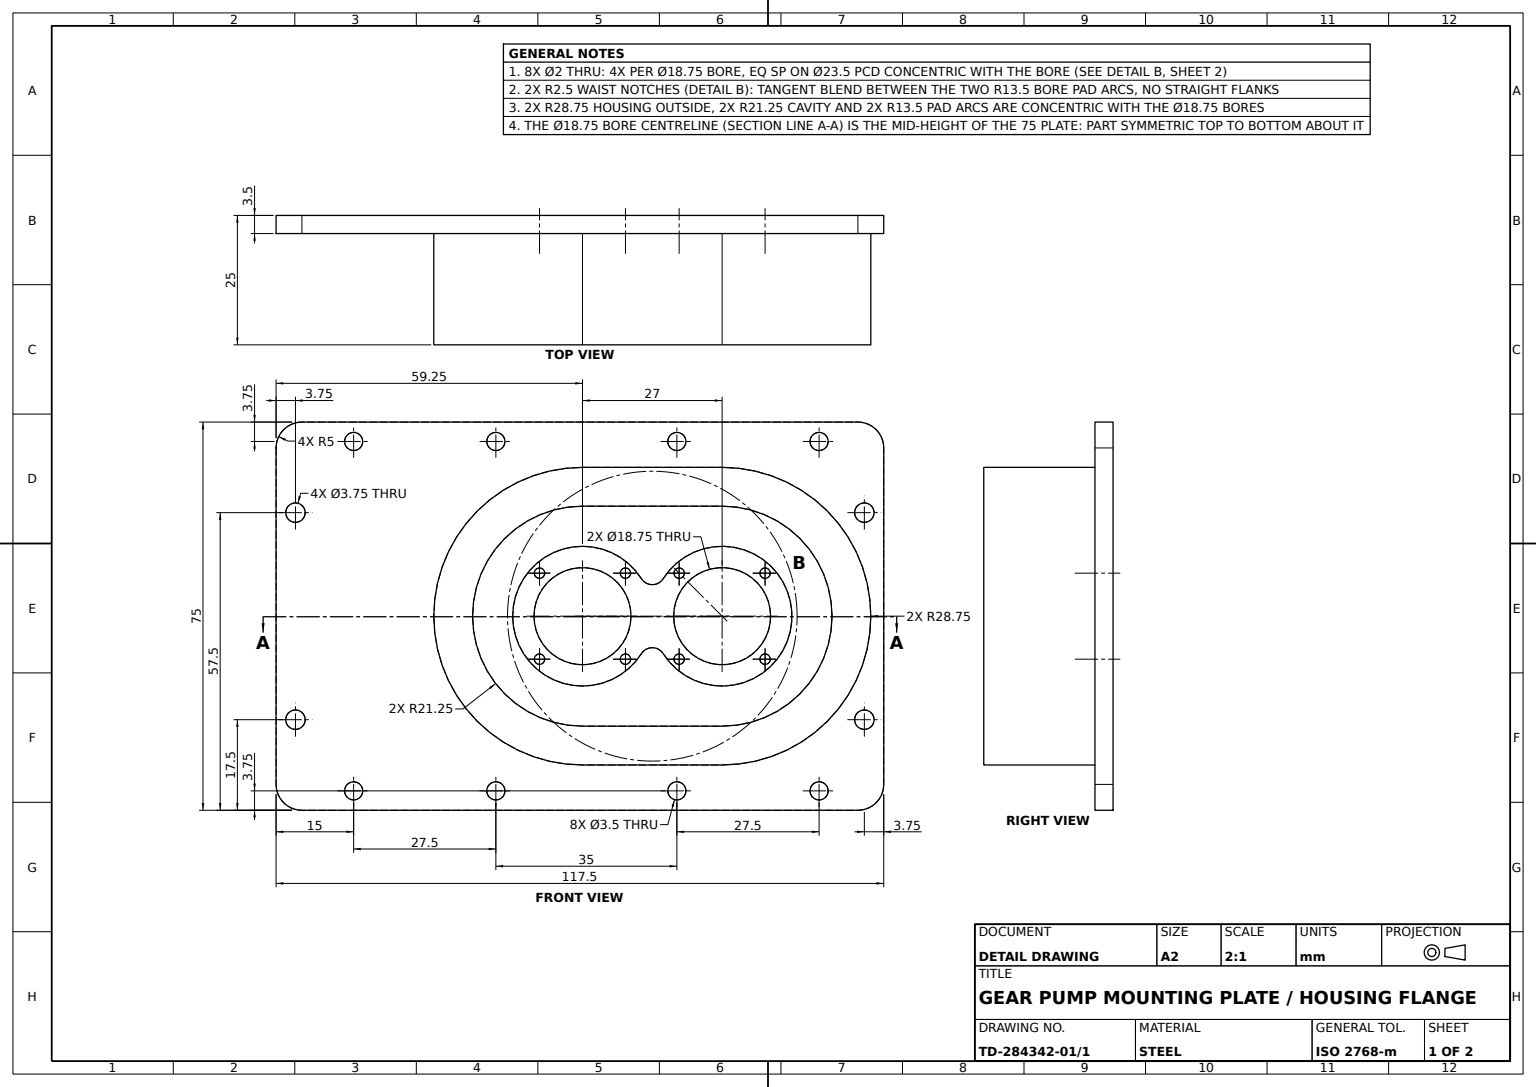
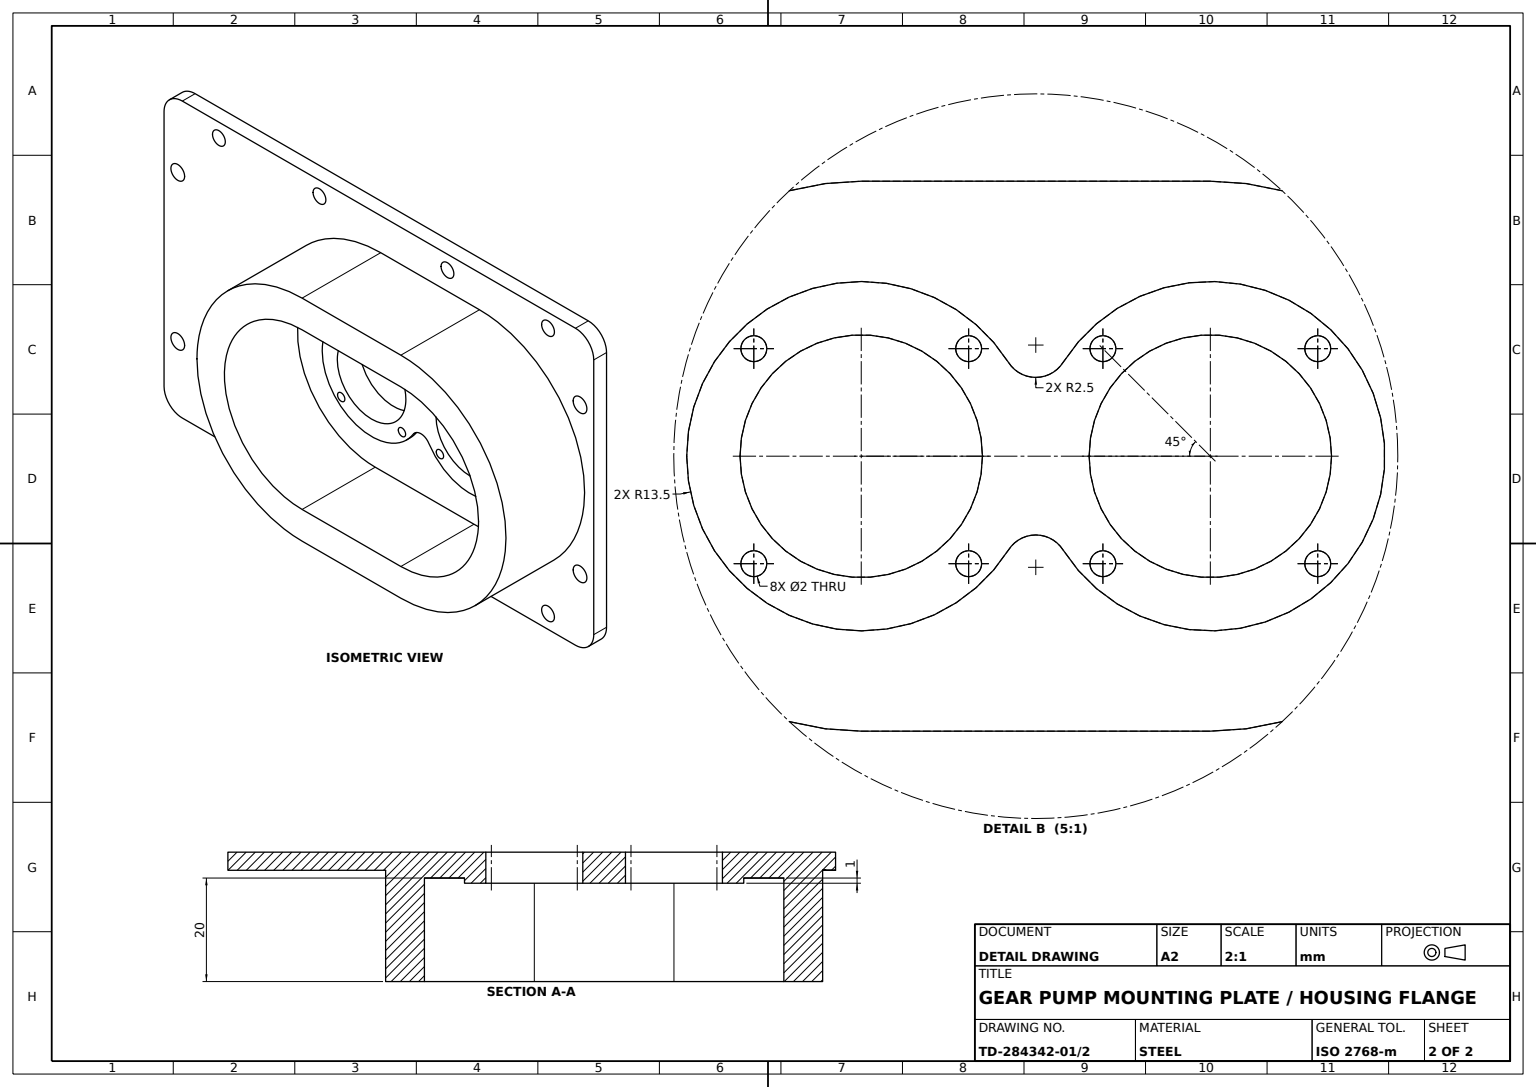
solid
v1 (86.25,8.75,25)
v2 (86.25,66.25,25)
e1 v1 v2 CIRCLE(AX(P(86.25,37.5,25),D(0,0,1),D(1,0,0)),28.75)
v3 (86.25,8.75,3.5)
e2 v1 v3 LINE
v4 (86.25,66.25,3.5)
e3 v3 v4 CIRCLE(AX(P(86.25,37.5,3.5),D(0,0,1),D(1,0,0)),28.75)
e4 v2 v4 LINE
face CYL(AX(P(86.25,37.5,25),D(0,0,-1),D(-1,0,0)),28.75) [-e1 e2 e3 -e4]
v5 (70.640625,44.745941,5)
v6 (45.75,37.5,5)
e5 v5 v6 CIRCLE(AX(P(59.25,37.5,5),D(0,0,1),D(1,0,0)),13.5)
v7 (45.75,37.5,6)
e6 v7 v6 LINE
v8 (70.640625,44.745941,6)
e7 v8 v7 CIRCLE(AX(P(59.25,37.5,6),D(0,0,1),D(1,0,0)),13.5)
e8 v8 v5 LINE
face CYL(AX(P(59.25,37.5,6),D(0,0,-1),D(-1,0,0)),13.5) [e5 -e6 -e7 e8]
v9 (40.75,3.75,3.5)
v10 (44.25,3.75,3.5)
e9 v9 v10 CIRCLE(AX(P(42.5,3.75,3.5),D(0,0,-1),D(1,0,0)),1.75)
v11 (40.75,3.75,0)
e10 v11 v9 LINE
v12 (44.25,3.75,0)
e11 v11 v12 CIRCLE(AX(P(42.5,3.75,0),D(0,0,-1),D(1,0,0)),1.75)
e12 v12 v10 LINE
face CYL(AX(P(42.5,3.75,0),D(0,0,1),D(1,0,0)),1.75) rev [-e9 -e10 e11 e12]
v13 (1.875,57.5,0)
v14 (1.875,57.5,3.5)
e13 v13 v14 LINE
v15 (5.625,57.5,0)
e14 v13 v15 CIRCLE(AX(P(3.75,57.5,0),D(0,0,-1),D(-1,0,0)),1.875)
v16 (5.625,57.5,3.5)
e15 v15 v16 LINE
e16 v14 v16 CIRCLE(AX(P(3.75,57.5,3.5),D(0,0,-1),D(-1,0,0)),1.875)
face CYL(AX(P(3.75,57.5,0),D(0,0,1),D(1,0,0)),1.875) rev [-e13 e14 e15 -e16]
v17 (74.859375,44.745941,5)
e17 v17 v5 CIRCLE(AX(P(72.75,46.087782,5),D(0,0,-1),D(1,0,0)),2.5)
v18 (74.859375,30.254059,5)
e18 v18 v17 CIRCLE(AX(P(86.25,37.5,5),D(0,0,1),D(1,0,0)),13.5)
v19 (70.640625,30.254059,5)
e19 v19 v18 CIRCLE(AX(P(72.75,28.912218,5),D(0,0,-1),D(1,0,0)),2.5)
e20 v6 v19 CIRCLE(AX(P(59.25,37.5,5),D(0,0,1),D(1,0,0)),13.5)
v20 (86.25,58.75,5)
v21 (59.25,58.75,5)
e21 v20 v21 LINE
v22 (59.25,16.25,5)
e22 v21 v22 CIRCLE(AX(P(59.25,37.5,5),D(0,0,1),D(1,0,0)),21.25)
v23 (86.25,16.25,5)
e23 v22 v23 LINE
v24 (107.5,37.5,5)
e24 v23 v24 CIRCLE(AX(P(86.25,37.5,5),D(0,0,1),D(1,0,0)),21.25)
e25 v24 v20 CIRCLE(AX(P(86.25,37.5,5),D(0,0,1),D(1,0,0)),21.25)
face PLANE(AX(P(86.25,37.5,5),D(0,0,1),D(1,0,0))) [-e17 -e18 -e19 -e20 -e5] [e21 e22 e23 e24 e25]
v25 (1.875,17.5,3.5)
v26 (5.625,17.5,3.5)
e26 v25 v26 CIRCLE(AX(P(3.75,17.5,3.5),D(0,0,-1),D(-1,0,0)),1.875)
v27 (1.875,17.5,0)
e27 v27 v25 LINE
v28 (5.625,17.5,0)
e28 v27 v28 CIRCLE(AX(P(3.75,17.5,0),D(0,0,-1),D(-1,0,0)),1.875)
e29 v28 v26 LINE
face CYL(AX(P(3.75,17.5,0),D(0,0,1),D(1,0,0)),1.875) rev [-e26 -e27 e28 e29]
v29 (103.25,71.25,0)
v30 (106.75,71.25,0)
e30 v29 v30 CIRCLE(AX(P(105,71.25,0),D(0,0,1),D(1,0,0)),1.75)
v31 (103.25,71.25,3.5)
e31 v29 v31 LINE
v32 (106.75,71.25,3.5)
e32 v31 v32 CIRCLE(AX(P(105,71.25,3.5),D(0,0,1),D(1,0,0)),1.75)
e33 v30 v32 LINE
face CYL(AX(P(105,71.25,0),D(0,0,1),D(1,0,0)),1.75) rev [-e30 e31 e32 -e33]
v33 (95.558505,29.191495,0)
v34 (95.558505,29.191495,6)
e34 v33 v34 LINE
v35 (93.558505,29.191495,0)
e35 v35 v33 CIRCLE(AX(P(94.558505,29.191495,0),D(0,0,1),D(1,0,0)),1)
v36 (93.558505,29.191495,6)
e36 v35 v36 LINE
e37 v36 v34 CIRCLE(AX(P(94.558505,29.191495,6),D(0,0,1),D(1,0,0)),1)
face CYL(AX(P(94.558505,29.191495,0),D(0,0,1),D(1,0,0)),1) rev [-e34 -e35 e36 e37]
v37 (79.25,3.75,0)
v38 (75.75,3.75,0)
e38 v37 v38 CIRCLE(AX(P(77.5,3.75,0),D(0,0,-1),D(1,0,0)),1.75)
v39 (75.75,3.75,3.5)
e39 v38 v39 LINE
v40 (79.25,3.75,3.5)
e40 v40 v39 CIRCLE(AX(P(77.5,3.75,3.5),D(0,0,-1),D(1,0,0)),1.75)
e41 v37 v40 LINE
face CYL(AX(P(77.5,3.75,0),D(0,0,1),D(1,0,0)),1.75) rev [e38 e39 -e40 -e41]
v41 (51.941495,29.191495,0)
v42 (51.941495,29.191495,6)
e42 v41 v42 LINE
v43 (49.941495,29.191495,0)
e43 v43 v41 CIRCLE(AX(P(50.941495,29.191495,0),D(0,0,1),D(0,-1,0)),1)
v44 (49.941495,29.191495,6)
e44 v43 v44 LINE
e45 v44 v42 CIRCLE(AX(P(50.941495,29.191495,6),D(0,0,1),D(0,-1,0)),1)
face CYL(AX(P(50.941495,29.191495,0),D(0,0,1),D(1,0,0)),1) rev [-e42 -e43 e44 e45]
v45 (117.5,5,0)
v46 (117.5,70,0)
e46 v45 v46 LINE
v47 (117.5,70,3.5)
e47 v46 v47 LINE
v48 (117.5,5,3.5)
e48 v48 v47 LINE
e49 v48 v45 LINE
face PLANE(AX(P(117.5,0,3.5),D(-1,0,0),D(0,0,1))) rev [e46 e47 -e48 e49]
v49 (44.25,71.25,3.5)
v50 (40.75,71.25,3.5)
e50 v49 v50 CIRCLE(AX(P(42.5,71.25,3.5),D(0,0,1),D(1,0,0)),1.75)
v51 (40.75,71.25,0)
e51 v51 v50 LINE
v52 (44.25,71.25,0)
e52 v52 v51 CIRCLE(AX(P(42.5,71.25,0),D(0,0,1),D(1,0,0)),1.75)
e53 v52 v49 LINE
face CYL(AX(P(42.5,71.25,0),D(0,0,1),D(1,0,0)),1.75) rev [e50 -e51 -e52 e53]
v53 (74.859375,44.745941,6)
e54 v53 v8 CIRCLE(AX(P(72.75,46.087782,6),D(0,0,-1),D(1,0,0)),2.5)
e55 v53 v17 LINE
face CYL(AX(P(72.75,46.087782,6),D(0,0,-1),D(-1,0,0)),2.5) rev [-e54 e55 e17 -e8]
v54 (68.625,37.5,0)
v55 (68.625,37.5,6)
e56 v54 v55 LINE
v56 (49.875,37.5,0)
e57 v56 v54 CIRCLE(AX(P(59.25,37.5,0),D(0,0,1),D(1,0,0)),9.375)
v57 (49.875,37.5,6)
e58 v56 v57 LINE
e59 v57 v55 CIRCLE(AX(P(59.25,37.5,6),D(0,0,1),D(1,0,0)),9.375)
face CYL(AX(P(59.25,37.5,0),D(0,0,1),D(1,0,0)),9.375) rev [-e56 -e57 e58 e59]
v58 (115.625,17.5,0)
v59 (115.625,17.5,3.5)
e60 v58 v59 LINE
v60 (111.875,17.5,3.5)
e61 v59 v60 CIRCLE(AX(P(113.75,17.5,3.5),D(0,0,1),D(1,0,0)),1.875)
v61 (111.875,17.5,0)
e62 v61 v60 LINE
e63 v58 v61 CIRCLE(AX(P(113.75,17.5,0),D(0,0,1),D(1,0,0)),1.875)
face CYL(AX(P(113.75,17.5,0),D(0,0,1),D(1,0,0)),1.875) rev [e60 e61 -e62 -e63]
v62 (93.558505,45.808505,6)
v63 (95.558505,45.808505,6)
e64 v62 v63 CIRCLE(AX(P(94.558505,45.808505,6),D(0,0,1),D(0,1,0)),1)
v64 (95.558505,45.808505,0)
e65 v64 v63 LINE
v65 (93.558505,45.808505,0)
e66 v65 v64 CIRCLE(AX(P(94.558505,45.808505,0),D(0,0,1),D(0,1,0)),1)
e67 v65 v62 LINE
face CYL(AX(P(94.558505,45.808505,0),D(0,0,1),D(1,0,0)),1) rev [e64 -e65 -e66 e67]
v66 (30.5,37.5,3.5)
v67 (59.25,8.75,3.5)
e68 v66 v67 CIRCLE(AX(P(59.25,37.5,3.5),D(0,0,1),D(1,0,0)),28.75)
v68 (59.25,8.75,25)
e69 v68 v67 LINE
v69 (30.5,37.5,25)
e70 v69 v68 CIRCLE(AX(P(59.25,37.5,25),D(0,0,1),D(1,0,0)),28.75)
e71 v69 v66 LINE
face CYL(AX(P(59.25,37.5,25),D(0,0,-1),D(-1,0,0)),28.75) [e68 -e69 -e70 e71]
v70 (95.625,37.5,6)
v71 (76.875,37.5,6)
e72 v70 v71 CIRCLE(AX(P(86.25,37.5,6),D(0,0,1),D(1,0,0)),9.375)
v72 (76.875,37.5,0)
e73 v72 v71 LINE
v73 (95.625,37.5,0)
e74 v73 v72 CIRCLE(AX(P(86.25,37.5,0),D(0,0,1),D(1,0,0)),9.375)
e75 v73 v70 LINE
face CYL(AX(P(86.25,37.5,0),D(0,0,1),D(1,0,0)),9.375) rev [e72 -e73 -e74 e75]
e76 v72 v73 CIRCLE(AX(P(86.25,37.5,0),D(0,0,1),D(1,0,0)),9.375)
e77 v71 v70 CIRCLE(AX(P(86.25,37.5,6),D(0,0,1),D(1,0,0)),9.375)
face CYL(AX(P(86.25,37.5,0),D(0,0,1),D(1,0,0)),9.375) rev [-e75 -e76 e73 e77]
v74 (107.5,37.5,25)
e78 v24 v74 LINE
v75 (86.25,58.75,25)
e79 v74 v75 CIRCLE(AX(P(86.25,37.5,25),D(0,0,1),D(1,0,0)),21.25)
e80 v20 v75 LINE
face CYL(AX(P(86.25,37.5,5),D(0,0,1),D(1,0,0)),21.25) rev [-e25 e78 e79 -e80]
v76 (70.640625,30.254059,6)
e81 v76 v19 LINE
e82 v7 v76 CIRCLE(AX(P(59.25,37.5,6),D(0,0,1),D(1,0,0)),13.5)
face CYL(AX(P(59.25,37.5,6),D(0,0,-1),D(-1,0,0)),13.5) [e20 -e81 -e82 e6]
v77 (59.25,16.25,25)
e83 v22 v77 LINE
v78 (86.25,16.25,25)
e84 v77 v78 LINE
e85 v23 v78 LINE
face PLANE(AX(P(86.25,16.25,5),D(0,-1,0),D(0,0,-1))) rev [-e23 e83 e84 -e85]
v79 (0,70,3.5)
v80 (0,70,0)
e86 v79 v80 LINE
v81 (0,5,0)
e87 v80 v81 LINE
v82 (0,5,3.5)
e88 v81 v82 LINE
e89 v79 v82 LINE
face PLANE(AX(P(0,75,3.5),D(1,0,0),D(0,0,-1))) rev [e86 e87 e88 -e89]
v83 (79.25,71.25,0)
v84 (79.25,71.25,3.5)
e90 v83 v84 LINE
v85 (75.75,71.25,3.5)
e91 v84 v85 CIRCLE(AX(P(77.5,71.25,3.5),D(0,0,1),D(1,0,0)),1.75)
v86 (75.75,71.25,0)
e92 v86 v85 LINE
e93 v83 v86 CIRCLE(AX(P(77.5,71.25,0),D(0,0,1),D(1,0,0)),1.75)
face CYL(AX(P(77.5,71.25,0),D(0,0,1),D(1,0,0)),1.75) rev [e90 e91 -e92 -e93]
v87 (5,0,0)
e94 v87 v81 CIRCLE(AX(P(5,5,0),D(0,0,-1),D(1,0,0)),5)
v88 (5,0,3.5)
e95 v88 v87 LINE
e96 v82 v88 CIRCLE(AX(P(5,5,3.5),D(0,0,1),D(1,0,0)),5)
face CYL(AX(P(5,5,3.5),D(0,0,-1),D(-1,0,0)),5) [-e88 -e94 -e95 -e96]
e97 v78 v74 CIRCLE(AX(P(86.25,37.5,25),D(0,0,1),D(1,0,0)),21.25)
face CYL(AX(P(86.25,37.5,5),D(0,0,1),D(1,0,0)),21.25) rev [e85 e97 -e78 -e24]
v89 (66.558505,29.191495,6)
v90 (68.558505,29.191495,6)
e98 v89 v90 CIRCLE(AX(P(67.558505,29.191495,6),D(0,0,1),D(1,0,0)),1)
v91 (68.558505,29.191495,0)
e99 v91 v90 LINE
v92 (66.558505,29.191495,0)
e100 v92 v91 CIRCLE(AX(P(67.558505,29.191495,0),D(0,0,1),D(1,0,0)),1)
e101 v92 v89 LINE
face CYL(AX(P(67.558505,29.191495,0),D(0,0,1),D(1,0,0)),1) rev [e98 -e99 -e100 e101]
e102 v34 v36 CIRCLE(AX(P(94.558505,29.191495,6),D(0,0,1),D(1,0,0)),1)
e103 v33 v35 CIRCLE(AX(P(94.558505,29.191495,0),D(0,0,1),D(1,0,0)),1)
face CYL(AX(P(94.558505,29.191495,0),D(0,0,1),D(1,0,0)),1) rev [e34 e102 -e36 -e103]
v93 (66.558505,45.808505,6)
v94 (68.558505,45.808505,6)
e104 v93 v94 CIRCLE(AX(P(67.558505,45.808505,6),D(0,0,1),D(0,1,0)),1)
v95 (68.558505,45.808505,0)
e105 v95 v94 LINE
v96 (66.558505,45.808505,0)
e106 v96 v95 CIRCLE(AX(P(67.558505,45.808505,0),D(0,0,1),D(0,1,0)),1)
e107 v96 v93 LINE
face CYL(AX(P(67.558505,45.808505,0),D(0,0,1),D(1,0,0)),1) rev [e104 -e105 -e106 e107]
v97 (13.25,71.25,0)
v98 (13.25,71.25,3.5)
e108 v97 v98 LINE
v99 (16.75,71.25,0)
e109 v99 v97 CIRCLE(AX(P(15,71.25,0),D(0,0,1),D(1,0,0)),1.75)
v100 (16.75,71.25,3.5)
e110 v99 v100 LINE
e111 v100 v98 CIRCLE(AX(P(15,71.25,3.5),D(0,0,1),D(1,0,0)),1.75)
face CYL(AX(P(15,71.25,0),D(0,0,1),D(1,0,0)),1.75) rev [-e108 -e109 e110 e111]
v101 (112.5,75,3.5)
v102 (112.5,75,0)
e112 v101 v102 LINE
e113 v47 v101 CIRCLE(AX(P(112.5,70,3.5),D(0,0,1),D(1,0,0)),5)
e114 v102 v46 CIRCLE(AX(P(112.5,70,0),D(0,0,-1),D(1,0,0)),5)
face CYL(AX(P(112.5,70,3.5),D(0,0,-1),D(-1,0,0)),5) [-e112 -e113 -e47 -e114]
v103 (76.941495,29.191495,0)
v104 (76.941495,29.191495,6)
e115 v103 v104 LINE
v105 (78.941495,29.191495,0)
e116 v105 v103 CIRCLE(AX(P(77.941495,29.191495,0),D(0,0,1),D(0,-1,0)),1)
v106 (78.941495,29.191495,6)
e117 v105 v106 LINE
e118 v106 v104 CIRCLE(AX(P(77.941495,29.191495,6),D(0,0,1),D(0,-1,0)),1)
face CYL(AX(P(77.941495,29.191495,0),D(0,0,1),D(1,0,0)),1) rev [-e115 -e116 e117 e118]
e119 v86 v83 CIRCLE(AX(P(77.5,71.25,0),D(0,0,1),D(1,0,0)),1.75)
e120 v28 v27 CIRCLE(AX(P(3.75,17.5,0),D(0,0,-1),D(-1,0,0)),1.875)
e121 v61 v58 CIRCLE(AX(P(113.75,17.5,0),D(0,0,1),D(1,0,0)),1.875)
e122 v95 v96 CIRCLE(AX(P(67.558505,45.808505,0),D(0,0,1),D(0,1,0)),1)
e123 v51 v52 CIRCLE(AX(P(42.5,71.25,0),D(0,0,1),D(1,0,0)),1.75)
e124 v12 v11 CIRCLE(AX(P(42.5,3.75,0),D(0,0,-1),D(1,0,0)),1.75)
v107 (16.75,3.75,0)
v108 (13.25,3.75,0)
e125 v107 v108 CIRCLE(AX(P(15,3.75,0),D(0,0,-1),D(1,0,0)),1.75)
e126 v108 v107 CIRCLE(AX(P(15,3.75,0),D(0,0,-1),D(1,0,0)),1.75)
v109 (112.5,0,0)
e127 v87 v109 LINE
v110 (5,75,0)
e128 v80 v110 CIRCLE(AX(P(5,70,0),D(0,0,-1),D(1,0,0)),5)
e129 v102 v110 LINE
e130 v45 v109 CIRCLE(AX(P(112.5,5,0),D(0,0,-1),D(1,0,0)),5)
v111 (106.75,3.75,0)
v112 (103.25,3.75,0)
e131 v111 v112 CIRCLE(AX(P(105,3.75,0),D(0,0,-1),D(1,0,0)),1.75)
e132 v112 v111 CIRCLE(AX(P(105,3.75,0),D(0,0,-1),D(1,0,0)),1.75)
e133 v15 v13 CIRCLE(AX(P(3.75,57.5,0),D(0,0,-1),D(-1,0,0)),1.875)
v113 (49.941495,45.808505,0)
v114 (51.941495,45.808505,0)
e134 v113 v114 CIRCLE(AX(P(50.941495,45.808505,0),D(0,0,1),D(-1,0,0)),1)
e135 v114 v113 CIRCLE(AX(P(50.941495,45.808505,0),D(0,0,1),D(-1,0,0)),1)
e136 v30 v29 CIRCLE(AX(P(105,71.25,0),D(0,0,1),D(1,0,0)),1.75)
e137 v38 v37 CIRCLE(AX(P(77.5,3.75,0),D(0,0,-1),D(1,0,0)),1.75)
e138 v103 v105 CIRCLE(AX(P(77.941495,29.191495,0),D(0,0,1),D(0,-1,0)),1)
e139 v97 v99 CIRCLE(AX(P(15,71.25,0),D(0,0,1),D(1,0,0)),1.75)
e140 v54 v56 CIRCLE(AX(P(59.25,37.5,0),D(0,0,1),D(1,0,0)),9.375)
e141 v41 v43 CIRCLE(AX(P(50.941495,29.191495,0),D(0,0,1),D(0,-1,0)),1)
e142 v91 v92 CIRCLE(AX(P(67.558505,29.191495,0),D(0,0,1),D(1,0,0)),1)
v115 (111.875,57.5,0)
v116 (115.625,57.5,0)
e143 v115 v116 CIRCLE(AX(P(113.75,57.5,0),D(0,0,1),D(1,0,0)),1.875)
e144 v116 v115 CIRCLE(AX(P(113.75,57.5,0),D(0,0,1),D(1,0,0)),1.875)
e145 v64 v65 CIRCLE(AX(P(94.558505,45.808505,0),D(0,0,1),D(0,1,0)),1)
v117 (76.941495,45.808505,0)
v118 (78.941495,45.808505,0)
e146 v117 v118 CIRCLE(AX(P(77.941495,45.808505,0),D(0,0,1),D(-1,0,0)),1)
e147 v118 v117 CIRCLE(AX(P(77.941495,45.808505,0),D(0,0,1),D(-1,0,0)),1)
face PLANE(AX(P(0,0,0),D(0,0,1),D(1,0,0))) rev [e93 e119] [-e28 -e120] [e121 e63] [e122 e106] [e52 e123] [-e11 -e124] [-e125 -e126] [e35 e103] [-e127 e94 -e87 e128 -e129 e114 -e46 e130] [-e131 -e132] [-e133 -e14] [e134 e135] [e136 e30] [-e38 -e137] [e116 e138] [e109 e139] [e140 e57] [e43 e141] [e142 e100] [e76 e74] [e143 e144] [e66 e145] [e146 e147]
e148 v60 v59 CIRCLE(AX(P(113.75,17.5,3.5),D(0,0,1),D(1,0,0)),1.875)
face CYL(AX(P(113.75,17.5,0),D(0,0,1),D(1,0,0)),1.875) rev [-e60 -e121 e62 e148]
v119 (74.859375,30.254059,6)
e149 v76 v119 CIRCLE(AX(P(72.75,28.912218,6),D(0,0,-1),D(1,0,0)),2.5)
e150 v119 v53 CIRCLE(AX(P(86.25,37.5,6),D(0,0,1),D(1,0,0)),13.5)
e151 v63 v62 CIRCLE(AX(P(94.558505,45.808505,6),D(0,0,1),D(0,1,0)),1)
e152 v94 v93 CIRCLE(AX(P(67.558505,45.808505,6),D(0,0,1),D(0,1,0)),1)
e153 v104 v106 CIRCLE(AX(P(77.941495,29.191495,6),D(0,0,1),D(0,-1,0)),1)
e154 v55 v57 CIRCLE(AX(P(59.25,37.5,6),D(0,0,1),D(1,0,0)),9.375)
e155 v90 v89 CIRCLE(AX(P(67.558505,29.191495,6),D(0,0,1),D(1,0,0)),1)
v120 (49.941495,45.808505,6)
v121 (51.941495,45.808505,6)
e156 v120 v121 CIRCLE(AX(P(50.941495,45.808505,6),D(0,0,1),D(-1,0,0)),1)
e157 v121 v120 CIRCLE(AX(P(50.941495,45.808505,6),D(0,0,1),D(-1,0,0)),1)
v122 (76.941495,45.808505,6)
v123 (78.941495,45.808505,6)
e158 v122 v123 CIRCLE(AX(P(77.941495,45.808505,6),D(0,0,1),D(-1,0,0)),1)
e159 v123 v122 CIRCLE(AX(P(77.941495,45.808505,6),D(0,0,1),D(-1,0,0)),1)
e160 v42 v44 CIRCLE(AX(P(50.941495,29.191495,6),D(0,0,1),D(0,-1,0)),1)
face PLANE(AX(P(79.5,41.793891,6),D(0,0,1),D(1,0,0))) [-e72 -e77] [e54 e7 e82 e149 e150] [-e64 -e151] [-e104 -e152] [-e153 -e118] [-e102 -e37] [-e154 -e59] [-e155 -e98] [-e156 -e157] [-e158 -e159] [-e45 -e160]
e161 v10 v9 CIRCLE(AX(P(42.5,3.75,3.5),D(0,0,-1),D(1,0,0)),1.75)
face CYL(AX(P(42.5,3.75,0),D(0,0,1),D(1,0,0)),1.75) rev [-e12 e124 e10 -e161]
e162 v113 v120 LINE
e163 v114 v121 LINE
face CYL(AX(P(50.941495,45.808505,0),D(0,0,1),D(1,0,0)),1) rev [e162 e156 -e163 -e134]
e164 v67 v3 LINE
e165 v68 v1 LINE
face PLANE(AX(P(59.25,8.75,25),D(0,1,0),D(0,0,1))) rev [e164 -e2 -e165 e69]
v124 (59.25,58.75,25)
e166 v21 v124 LINE
e167 v124 v77 CIRCLE(AX(P(59.25,37.5,25),D(0,0,1),D(1,0,0)),21.25)
face CYL(AX(P(59.25,37.5,5),D(0,0,1),D(1,0,0)),21.25) rev [-e83 -e22 e166 e167]
e168 v26 v25 CIRCLE(AX(P(3.75,17.5,3.5),D(0,0,-1),D(-1,0,0)),1.875)
face CYL(AX(P(3.75,17.5,0),D(0,0,1),D(1,0,0)),1.875) rev [-e168 -e29 e120 e27]
e169 v39 v40 CIRCLE(AX(P(77.5,3.75,3.5),D(0,0,-1),D(1,0,0)),1.75)
face CYL(AX(P(77.5,3.75,0),D(0,0,1),D(1,0,0)),1.75) rev [-e169 -e39 e137 e41]
v125 (112.5,0,3.5)
e170 v109 v125 LINE
e171 v125 v48 CIRCLE(AX(P(112.5,5,3.5),D(0,0,1),D(1,0,0)),5)
face CYL(AX(P(112.5,5,3.5),D(0,0,-1),D(-1,0,0)),5) [-e170 -e130 -e49 -e171]
face CYL(AX(P(77.941495,29.191495,0),D(0,0,1),D(1,0,0)),1) rev [e115 e153 -e117 -e138]
v126 (111.875,57.5,3.5)
e172 v115 v126 LINE
v127 (115.625,57.5,3.5)
e173 v116 v127 LINE
e174 v127 v126 CIRCLE(AX(P(113.75,57.5,3.5),D(0,0,1),D(1,0,0)),1.875)
face CYL(AX(P(113.75,57.5,0),D(0,0,1),D(1,0,0)),1.875) rev [-e172 -e144 e173 e174]
e175 v119 v18 LINE
face CYL(AX(P(86.25,37.5,6),D(0,0,-1),D(-1,0,0)),13.5) [e175 e18 -e55 -e150]
e176 v32 v31 CIRCLE(AX(P(105,71.25,3.5),D(0,0,1),D(1,0,0)),1.75)
face CYL(AX(P(105,71.25,0),D(0,0,1),D(1,0,0)),1.75) rev [e176 -e31 -e136 e33]
v128 (106.75,3.75,3.5)
e177 v111 v128 LINE
v129 (103.25,3.75,3.5)
e178 v112 v129 LINE
e179 v128 v129 CIRCLE(AX(P(105,3.75,3.5),D(0,0,-1),D(1,0,0)),1.75)
face CYL(AX(P(105,3.75,0),D(0,0,1),D(1,0,0)),1.75) rev [-e177 e131 e178 -e179]
e180 v129 v128 CIRCLE(AX(P(105,3.75,3.5),D(0,0,-1),D(1,0,0)),1.75)
face CYL(AX(P(105,3.75,0),D(0,0,1),D(1,0,0)),1.75) rev [-e180 -e178 e132 e177]
e181 v75 v124 LINE
v130 (59.25,66.25,25)
e182 v130 v69 CIRCLE(AX(P(59.25,37.5,25),D(0,0,1),D(1,0,0)),28.75)
e183 v2 v130 LINE
face PLANE(AX(P(59.25,37.5,25),D(0,0,1),D(1,0,0))) [-e97 -e84 -e167 -e181 -e79] [e182 e70 e165 e1 e183]
v131 (13.25,3.75,3.5)
e184 v108 v131 LINE
v132 (16.75,3.75,3.5)
e185 v132 v131 CIRCLE(AX(P(15,3.75,3.5),D(0,0,-1),D(1,0,0)),1.75)
e186 v107 v132 LINE
face CYL(AX(P(15,3.75,0),D(0,0,1),D(1,0,0)),1.75) rev [e125 e184 -e185 -e186]
e187 v117 v122 LINE
e188 v118 v123 LINE
face CYL(AX(P(77.941495,45.808505,0),D(0,0,1),D(1,0,0)),1) rev [e159 -e187 -e147 e188]
v133 (5,75,3.5)
e189 v133 v79 CIRCLE(AX(P(5,70,3.5),D(0,0,1),D(1,0,0)),5)
e190 v110 v133 LINE
face CYL(AX(P(5,70,3.5),D(0,0,-1),D(-1,0,0)),5) [-e189 -e190 -e128 -e86]
e191 v16 v14 CIRCLE(AX(P(3.75,57.5,3.5),D(0,0,-1),D(-1,0,0)),1.875)
face CYL(AX(P(3.75,57.5,0),D(0,0,1),D(1,0,0)),1.875) rev [-e15 e133 e13 -e191]
face CYL(AX(P(72.75,28.912218,6),D(0,0,-1),D(-1,0,0)),2.5) rev [-e175 -e149 e81 e19]
v134 (59.25,66.25,3.5)
e192 v130 v134 LINE
e193 v134 v66 CIRCLE(AX(P(59.25,37.5,3.5),D(0,0,1),D(1,0,0)),28.75)
face CYL(AX(P(59.25,37.5,25),D(0,0,-1),D(-1,0,0)),28.75) [e192 e193 -e71 -e182]
e194 v101 v133 LINE
face PLANE(AX(P(117.5,75,3.5),D(0,-1,0),D(0,0,-1))) rev [e190 -e194 e112 e129]
face CYL(AX(P(77.941495,45.808505,0),D(0,0,1),D(1,0,0)),1) rev [e158 -e188 -e146 e187]
e195 v98 v100 CIRCLE(AX(P(15,71.25,3.5),D(0,0,1),D(1,0,0)),1.75)
face CYL(AX(P(15,71.25,0),D(0,0,1),D(1,0,0)),1.75) rev [-e139 e108 e195 -e110]
face PLANE(AX(P(86.25,58.75,5),D(0,1,0),D(0,0,1))) rev [-e21 e80 e181 -e166]
face CYL(AX(P(50.941495,45.808505,0),D(0,0,1),D(1,0,0)),1) rev [-e162 -e135 e163 e157]
e196 v50 v49 CIRCLE(AX(P(42.5,71.25,3.5),D(0,0,1),D(1,0,0)),1.75)
face CYL(AX(P(42.5,71.25,0),D(0,0,1),D(1,0,0)),1.75) rev [e51 e196 -e53 -e123]
face CYL(AX(P(94.558505,45.808505,0),D(0,0,1),D(1,0,0)),1) rev [-e67 -e145 e65 e151]
e197 v4 v134 LINE
face PLANE(AX(P(59.25,66.25,25),D(0,-1,0),D(0,0,-1))) rev [-e192 -e183 e4 e197]
face CYL(AX(P(59.25,37.5,0),D(0,0,1),D(1,0,0)),9.375) rev [e56 e154 -e58 -e140]
e198 v131 v132 CIRCLE(AX(P(15,3.75,3.5),D(0,0,-1),D(1,0,0)),1.75)
face CYL(AX(P(15,3.75,0),D(0,0,1),D(1,0,0)),1.75) rev [e186 -e198 -e184 e126]
e199 v126 v127 CIRCLE(AX(P(113.75,57.5,3.5),D(0,0,1),D(1,0,0)),1.875)
e200 v85 v84 CIRCLE(AX(P(77.5,71.25,3.5),D(0,0,1),D(1,0,0)),1.75)
e201 v88 v125 LINE
face PLANE(AX(P(0,0,3.5),D(0,0,1),D(1,0,0))) [e9 e161] [-e50 -e196] [-e148 -e61] [e26 e168] [-e176 -e32] [e191 e16] [-e174 -e199] [-e68 -e193 -e197 -e3 -e164] [e169 e40] [e185 e198] [-e111 -e195] [e180 e179] [-e200 -e91] [e89 e96 e201 e171 e48 e113 e194 e189]
face CYL(AX(P(67.558505,29.191495,0),D(0,0,1),D(1,0,0)),1) rev [-e101 -e142 e99 e155]
face CYL(AX(P(67.558505,45.808505,0),D(0,0,1),D(1,0,0)),1) rev [e152 -e107 -e122 e105]
face CYL(AX(P(50.941495,29.191495,0),D(0,0,1),D(1,0,0)),1) rev [e42 e160 -e44 -e141]
face PLANE(AX(P(0,0,3.5),D(0,1,0),D(0,0,1))) rev [e170 -e201 e95 e127]
face CYL(AX(P(113.75,57.5,0),D(0,0,1),D(1,0,0)),1.875) rev [-e173 -e143 e172 e199]
face CYL(AX(P(77.5,71.25,0),D(0,0,1),D(1,0,0)),1.75) rev [e200 -e90 -e119 e92]
